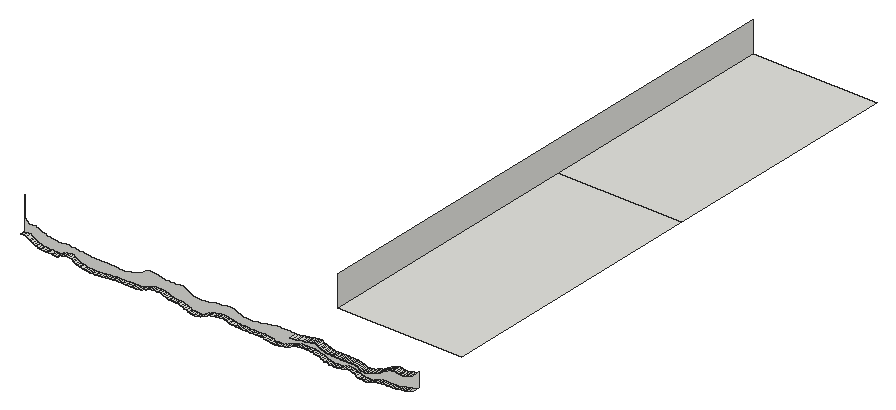
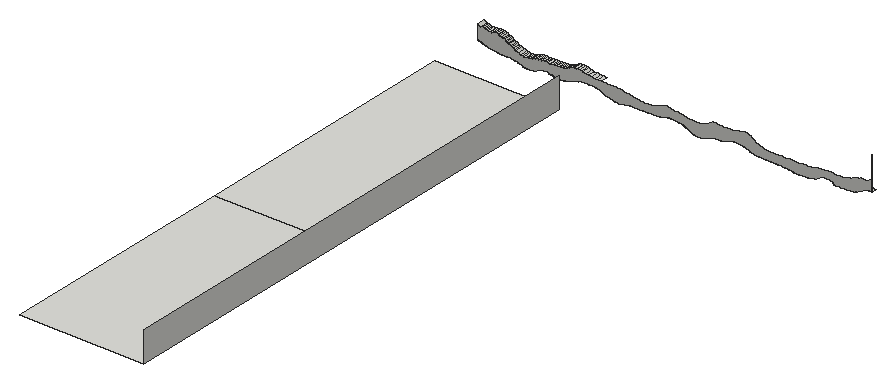
# SketchUp Ruby script. Lengths in inches.
U = 1.inch
M = Sketchup.active_model
def pt(a) = Geom::Point3d.new(a.map { |v| v * U })
def face(e, loops, mat)
  f = e.add_face(loops[0].map { |a| pt(a) })
  loops[1..].each { |l| e.add_face(l.map { |a| pt(a) }).erase! }
  f.material = f.back_material = mat if mat
  f
end
# faces: each face lists its corners as indices into pts; further lists are holes
def faces(e, pts, list, mat = nil) = list.each { |f| face(e, (f[0].is_a?(Array) ? f : [f]).map { |l| l.map { |i| pts[i] } }, mat) }
# xy, xz, yz: faces in a plane at the given z, y or x. An outline is a flat list of corners, or four numbers for a rectangle; further outlines are holes
def ring(l) = l.size == 4 ? [[l[0], l[1]], [l[2], l[1]], [l[2], l[3]], [l[0], l[3]]] : l.each_slice(2).to_a
def flat(e, list, mat, &to3) = list.each { |f| face(e, (f[0].is_a?(Array) ? f : [f]).map { |l| ring(l).map { |u, v| to3.(u, v) } }, mat) }
def xy(e, z, list, mat = nil) = flat(e, list, mat) { |x, y| [x, y, z] }
def xz(e, y, list, mat = nil) = flat(e, list, mat) { |x, z| [x, y, z] }
def yz(e, x, list, mat = nil) = flat(e, list, mat) { |y, z| [x, y, z] }
def lines(e, pts, list) = list.each { |a, b| e.add_line(pt(pts[a]), pt(pts[b])) }
# prism: a flat outline (further loops are holes) pulled along v
def prism(e, loops, v, mat = nil)
  f = face(e, loops, mat); d = Geom::Vector3d.new(v.map { |x| x * U })
  f.pushpull(f.normal.samedirection?(d) ? d.length : -d.length)
end
def box(e, o, s, mat = nil) = prism(e, [[o, [o[0] + s[0], o[1], o[2]], [o[0] + s[0], o[1] + s[1], o[2]], [o[0], o[1] + s[1], o[2]]]], [0, 0, s[2]], mat)
def at(x, y, z, deg = 0) = Geom::Transformation.translation(pt([x, y, z])) * Geom::Transformation.rotation(ORIGIN, Z_AXIS, deg.degrees)
def axes(o, x, y, z) = Geom::Transformation.new([*x, 0, *y, 0, *z, 0, *pt(o).to_a, 1])
def part(name) = M.definitions.add(name)
# library, detail: a bought-in or finely detailed component or shape, given as its bounding box
def library(name, o, s) = part(name).tap { |d| box(d.entities, o, s) }
def detail(e, o, s) = box(e.add_group.entities, o, s)
def put(e, d, t, mat = nil) = e.add_instance(d, t).tap { |i| i.material = mat if mat }
def group(e, t, mat = nil) = e.add_group.tap { |g| g.transformation = t; g.material = mat if mat }.entities
root = M.entities
xy(root,237.65,[[282.08,2402.3,282.77,2404.3],[282.77,2402.3,283.39,2404.3]])
xy(root,238.18,[[376.03,2402.3,376.71,2404.3]])
xy(root,238.33,[[291.18,2402.3,291.73,2404.3],[291.73,2402.3,292.41,2404.3]])
xy(root,238.34,[[293.09,2402.3,294.02,2404.3],[294.02,2402.3,294.51,2404.3],[294.51,2402.3,295.27,2404.3],[295.27,2402.3,295.9,2404.3],[295.9,2402.3,296.65,2404.3],
  [296.65,2402.3,297.27,2404.3],[297.27,2402.3,298.04,2404.3],[298.04,2402.3,298.66,2404.3]])
xy(root,238.62,[[342.56,2402.3,343.33,2404.3],[343.33,2402.3,343.96,2404.3],[343.96,2402.3,344.72,2404.3],[344.72,2402.3,345.34,2404.3],[345.34,2402.3,346.19,2404.3],
  [346.19,2402.3,346.83,2404.3],[346.83,2402.3,347.45,2404.3]])
xy(root,238.625,[[341.14,2402.3,342,2404.3]])
xy(root,238.89,[[396.95,2402.3,397.63,2404.3]])
xy(root,238.9,[[398.39,2402.3,399.01,2404.3],[399.01,2402.3,399.78,2404.3]])
xy(root,240.43,[[365.23,2402.3,365.8,2404.3]])
xy(root,241.52,[[252.78,2402.3,252.84,2404.3]])
xy(root,242.28,[[383.05,2401.37,383.5625,2404.3]])
xy(root,242.3,[[381.29,2401.37,381.96,2404.3]])
xy(root,242.33,[[378.88,2401.37,379.46,2404.3]])
xy(root,242.625,[[358.39,2425.46,406.85,2532.83],[358.39,2532.83,406.85,2628.15]])
xz(root,2404.3,[[321.7,236.98,321.09,237.01,320.4,237.04,319.64,237.11,318.95,237.2,318.42,237.33,317.75,237.68,316.8125,237.96,316.25,238.28,315.47,238.43,314.69,238.78,314.02,238.79,313.48,238.8,312.72,238.83,311.97,238.875,311.4,238.94,310.82,239.04,310.16,239.29,309.58,239.53,309.05,239.7,308.36,239.92,307.73,240.11,306.95,240.27,306.33,240.25,305.625,240.23,304.86,240.19,304.1875,240.12,303.53,240.03,302.89,239.85,302.34,239.52,301.78,239.35,301.19,239.18,300.68,238.86,299.99,238.72,299.17,238.59,298.66,238.34,293.09,238.34,292.41,238.33,291.18,238.33,290.46,238.32,289.61,238.3,288.98,238.28,288.23,238.26,287.6,238.15,286.84,238.13,286.29,238.1,285.4375,237.98,284.82,237.94,284.06,237.89,283.39,237.65,282.08,237.65,281.39,237.66,280.64,237.67,280.04,237.68,279.43,237.71,278.72,237.76,278.03,237.82,277.37,237.9,276.43,238.21,275.96,238.31,275.05,238.43,274.4,238.74,273.82,239.11,273.24,239.38,272.78,239.71,272.08,240.11,271.39,240.09,270.73,240.05,270.14,239.99,269.41,239.88,268.86,239.69,268.28,239.55,267.72,238.9375,267.19,238.77,266.45,238.79,265.58,238.8,265.07,238.82,264.03,238.92,263.34,238.93,262.64,238.94,261.94,238.97,261.26,239.03,260.57,239.09,259.79,239.19,259.28,239.52,258.72,239.64,258.27,239.86,257.48,240.2,256.88,240.59,256.34,240.85,255.32,241.55,254.05,241.69,252.84,241.52,252.84,246.2,254.41,244.96,255.8,244.9375,257.05,244.92,257.27,244.61,257.83,244.54,258.59,244.41,259.26,244.11,259.78,243.95,260.44,243.79,260.96,243.48,261.6,243.3,262.1875,243.14,262.67,243.06,263.39,242.85,263.97,242.78,264.78,242.73,265.32,242.68,265.99,242.51,266.51,242.46,267.05,242.58,267.68,242.57,268.31,242.81,268.88,242.86,269.44,242.89,270.08,242.92,270.51,242.625,271.12,242.65,271.67,242.62,272.3,242.58,272.86,242.57,273.5,242.48,274.16,242.38,274.82,242.34,275.49,242.24,276.66,241.96,277.43,241.89,278.25,241.83,278.85,241.78,279.62,241.75,280.07,241.74,280.62,241.72,281.88,241.7,282.61,241.69,283.28,241.68,283.87,241.68,284.36,241.67,285.0625,241.74,285.63,241.75,287.63,241.75,288.12,241.67,288.65,241.66,289.26,241.57,289.8,241.53,290.42,241.51,290.97,241.49,291.67,241.48,292.33,241.47,292.9,241.46,293.61,241.6,294.34,241.85,295.01,241.91,295.91,242.1,296.68,242.46,297.38,242.78,298.15,242.97,298.68,243.23,299.08,243.48,299.6,243.72,299.9375,244.12,300.41,244.39,300.89,244.73,301.375,244.87,301.96,244.95,302.64,245.01,303.29,244.81,303.86,244.7,304.34,244.67,304.95,244.55,305.49,244.51,305.95,244.25,306.7,244.11,307.26,244.04,307.88,243.99,308.6,243.95,309.1,243.93,309.79,243.91,310.36,243.89,311.06,243.88,311.71,243.94,312.35,243.95,312.91,244.1,313.54,244.13,314.02,244.15,314.54,244.17,315.06,244.18,315.66,243.8,316.2,243.43,316.81,243.09,317.2,242.875,317.7,242.68,318.29,242.51,318.8,242.21,319.4,242.11,320.08,241.96,320.64,241.89,321.1,241.85,321.62,241.8125,322.13,241.79,322.71,241.78,323.38,241.91,323.85,241.93,324.52,242.09,325.29,242.2,325.79,242.24,326.4,242.42,326.95,242.47,327.7,242.71,328.34,242.78,328.82,242.82,329.51,242.85,330.21,242.87,330.76,243.02,331.38,243.05,331.93,243.29,332.61,243.35,333.16,243.39,333.76,243.42,334.53,243.14,335.1,242.9375,335.65,242.65,336.27,242.39,337.03,242.14,337.67,241.89,338.16,241.78,339.21,241.63,339.98,241.56,340.58,241.51,341.03,241.48,341.55,241.46,342.42,241.51,343.14,241.59,344.08,241.82,344.86,241.87,345.625,241.98,346.24,242.02,346.89,242.19,347.59,242.38,348.08,242.4375,348.6,242.48,349.26,242.58,349.79,242.61,350.375,242.77,350.83,242.95,351.39,243.01,351.9,243.05,352.47,243.08,353.125,243.09,355.28,243.09,355.85,243.08,356.4375,243.07,357.02,243.07,357.68,243.0625,358.29,243.05,358.97,243.05,360.24,243.1,361.41,243.17,362.55,243.4,363.8125,243.52,364.94,243.71,365.84,243.99,366.54,244.08,367.24,244.21,367.82,244.27,368.36,244.3,369.03,244.39,369.625,244.19,370,243.88,370.48,243.59,371.03,243.33,371.58,243.22,372.07,242.92,372.55,242.75,373.11,242.6,373.67,242.52,374.23,242.47,374.8125,242.43,375.39,242.4,375.97,242.39,376.55,242.37,377.13,242.36,377.72,242.35,378.88,242.33,379.46,242.33,380.18,242.32,380.65,242.3125,381.29,242.3,381.96,242.3,382.41,242.29,383.05,242.28,383.5625,242.28,384.19,242.2,384.77,241.97,385.34,241.84,385.85,241.57,386.27,241.33,386.74,241.24,387.27,241.17,387.74,241.12,388.34,241.09,388.91,241.14,389.55,241.35,390.14,241.46,391.08,241.85,392.08,242.23,392.64,242.42,393.36,242.61,393.875,242.91,394.25,243.14,394.79,243.52,395.27,243.71,395.6,244.02,396.04,244.21,396.63,244.57,397.1,244.76,397.72,245.125,398.22,245.32,398.7,245.41,399.25,245.48,399.74,245.59,400.27,245.55,400.88,245.35,401.37,245.31,401.92,245.27,402.48,245.24,403.04,245.22,403.6,245.34,404.23,245.42,404.8125,245.52,405.19,245.76,405.66,245.9,406.85,246.43,406.85,240.89,405.02,240.1,404.46,239.96,403.9375,239.81,403.25,239.53,402.7,239.49,401.98,239.42,401.18,239.28,400.41,239.15,399.78,238.9,398.39,238.9,397.63,238.89,396.95,238.89,396.27,238.88,395.73,238.875,394.97,238.86,394.23,238.83,393.66,238.8,393.08,238.74,392.42,238.6,391.85,238.51,391.32,238.33,390.63,238.08,389.95,237.84,389.26,237.5625,388.66,237.47,387.98,237.4,387.25,237.42,386.68,237.45,386.09,237.51,385.49,237.59,384.95,237.71,384.12,238,383.41,238.33,382.86,238.57,382.36,238.86,381.84,238.96,381.15,239.02,380.47,239.125,379.73,239.04,379.16,238.66,378.57,238.61,377.91,238.55,377.39,238.27,376.71,238.18,376.03,238.18,375.36,238.11,374.83,238.15,374.01,238.19,373.4375,238.26,372.87,238.48,372.21,238.56,371.64,238.67,371.12,239.01,370.4375,239.18,369.8125,239.5,369.05,239.65,368.4375,239.8,367.68,239.96,367.03,240.23,366.45,240.27,365.8,240.43,365.23,240.43,364.65,240.42,364.125,240.41,363.43,240.4,362.74,240.37,362.05,240.33,361.37,240.27,360.69,240.17,360.07,239.97,359.42,239.75,358.68,239.375,357.89,239.08,357.01,238.72,356.26,238.46,355.04,238.14,353.92,237.88,353.27,237.87,352.4,237.74,351.69,237.79,350.92,237.86,350.29,238.15,349.52,238.19,348.9,238.25,348.14,238.45,347.45,238.62,342.56,238.62,342,238.625,341.14,238.625,340.45,238.63,339.83,238.64,339.05,238.65,338.38,238.66,337.69,238.6875,337.02,238.73,336.54,238.78,335.66,238.93,334.89,239.07,334.34,239.16,333.49,239.44,332.82,239.56,332.21,239.72,331.48,239.7,330.92,239.69,330.33,239.65,329.71,239.6,329.22,239.54,328.41,239.31,327.41,239.22,326.83,239.12,326.1875,238.76,325.55,238.51,324.99,238.375,324.55,238.02,323.85,237.74,323.23,237.43,322.38,237.22],[252.78,241.52,252.84,254.5]])
yz(root,358.39,[[2425.46,242.625,2628.15,254.5]])
p = [[319.64,2404.3,237.11],[320.4,2404.3,237.04],[320.4,2402.3,237.04],[319.64,2402.3,237.11],[321.09,2404.3,237.01],[321.09,2402.3,237.01],
  [321.7,2404.3,236.98],[321.7,2402.3,236.98],[322.38,2404.3,237.22],[322.38,2402.3,237.22],[318.95,2404.3,237.2],[318.95,2402.3,237.2],
  [318.42,2404.3,237.33],[318.42,2402.3,237.33],[323.23,2404.3,237.43],[323.23,2402.3,237.43],[317.75,2404.3,237.68],[317.75,2402.3,237.68],
  [323.85,2404.3,237.74],[323.85,2402.3,237.74],[386.68,2404.3,237.45],[387.25,2404.3,237.42],[387.25,2402.3,237.42],[386.68,2402.3,237.45],
  [387.98,2404.3,237.4],[387.98,2402.3,237.4],[388.66,2404.3,237.47],[388.66,2402.3,237.47],[385.49,2404.3,237.59],[386.09,2404.3,237.51],
  [386.09,2402.3,237.51],[385.49,2402.3,237.59],[389.26,2404.3,237.5625],[389.26,2402.3,237.5625],[283.39,2404.3,237.65],[284.06,2404.3,237.89],
  [284.06,2402.3,237.89],[283.39,2402.3,237.65],[384.95,2404.3,237.71],[384.95,2402.3,237.71],[389.95,2404.3,237.84],[389.95,2402.3,237.84],
  [278.72,2404.3,237.76],[279.43,2404.3,237.71],[279.43,2402.3,237.71],[278.72,2402.3,237.76],[280.04,2404.3,237.68],[280.04,2402.3,237.68],
  [280.64,2404.3,237.67],[280.64,2402.3,237.67],[281.39,2404.3,237.66],[281.39,2402.3,237.66],[282.08,2404.3,237.65],[282.08,2402.3,237.65],
  [316.8125,2404.3,237.96],[316.8125,2402.3,237.96],[324.55,2404.3,238.02],[324.55,2402.3,238.02],[351.69,2404.3,237.79],[352.4,2404.3,237.74],
  [352.4,2402.3,237.74],[351.69,2402.3,237.79],[353.27,2404.3,237.87],[353.27,2402.3,237.87],[384.12,2404.3,238],[384.12,2402.3,238],
  [277.37,2404.3,237.9],[278.03,2404.3,237.82],[278.03,2402.3,237.82],[277.37,2402.3,237.9],[350.92,2404.3,237.86],[350.92,2402.3,237.86],
  [390.63,2404.3,238.08],[390.63,2402.3,238.08],[276.43,2404.3,238.21],[276.43,2402.3,238.21],[284.82,2404.3,237.94],[284.82,2402.3,237.94],
  [285.4375,2404.3,237.98],[285.4375,2402.3,237.98],[350.29,2404.3,238.15],[350.29,2402.3,238.15],[353.92,2404.3,237.88],[353.92,2402.3,237.88],
  [355.04,2404.3,238.14],[355.04,2402.3,238.14],[286.29,2404.3,238.1],[286.29,2402.3,238.1],[316.25,2404.3,238.28],[316.25,2402.3,238.28],
  [324.99,2404.3,238.375],[324.99,2402.3,238.375],[383.41,2404.3,238.33],[383.41,2402.3,238.33],[286.84,2404.3,238.13],[286.84,2402.3,238.13],
  [287.6,2404.3,238.15],[287.6,2402.3,238.15],[349.52,2404.3,238.19],[349.52,2402.3,238.19],[356.26,2404.3,238.46],[356.26,2402.3,238.46],
  [374.01,2404.3,238.19],[374.83,2404.3,238.15],[374.83,2402.3,238.15],[374.01,2402.3,238.19],[375.36,2404.3,238.11],[375.36,2402.3,238.11],
  [376.03,2404.3,238.18],[376.03,2402.3,238.18],[391.32,2404.3,238.33],[391.32,2402.3,238.33],[275.96,2404.3,238.31],[275.96,2402.3,238.31],
  [288.23,2404.3,238.26],[288.23,2402.3,238.26],[348.9,2404.3,238.25],[348.9,2402.3,238.25],[373.4375,2404.3,238.26],[373.4375,2402.3,238.26],
  [376.71,2404.3,238.18],[377.39,2404.3,238.27],[377.39,2402.3,238.27],[376.71,2402.3,238.18],[275.05,2404.3,238.43],[275.05,2402.3,238.43],
  [288.98,2404.3,238.28],[288.98,2402.3,238.28],[289.61,2404.3,238.3],[289.61,2402.3,238.3],[290.46,2404.3,238.32],[290.46,2402.3,238.32],
  [291.18,2404.3,238.33],[291.18,2402.3,238.33],[292.41,2404.3,238.33],[293.09,2404.3,238.34],[293.09,2402.3,238.34],[292.41,2402.3,238.33],
  [298.66,2404.3,238.34],[299.17,2404.3,238.59],[299.17,2402.3,238.59],[298.66,2402.3,238.34],[315.47,2404.3,238.43],[315.47,2402.3,238.43],
  [348.14,2404.3,238.45],[348.14,2402.3,238.45],[372.87,2404.3,238.48],[372.87,2402.3,238.48],[377.91,2404.3,238.55],[377.91,2402.3,238.55],
  [382.86,2404.3,238.57],[382.86,2402.3,238.57],[391.85,2404.3,238.51],[391.85,2402.3,238.51],[274.4,2404.3,238.74],[274.4,2402.3,238.74],
  [314.69,2404.3,238.78],[314.69,2402.3,238.78],[325.55,2404.3,238.51],[325.55,2402.3,238.51],[326.1875,2404.3,238.76],[326.1875,2402.3,238.76],
  [347.45,2404.3,238.62],[347.45,2402.3,238.62],[357.01,2404.3,238.72],[357.01,2402.3,238.72],[372.21,2404.3,238.56],[372.21,2402.3,238.56],
  [378.57,2404.3,238.61],[378.57,2402.3,238.61],[392.42,2404.3,238.6],[392.42,2402.3,238.6],[299.99,2404.3,238.72],[299.99,2402.3,238.72],
  [338.38,2404.3,238.66],[339.05,2404.3,238.65],[339.05,2402.3,238.65],[338.38,2402.3,238.66],[339.83,2404.3,238.64],[339.83,2402.3,238.64],
  [340.45,2404.3,238.63],[340.45,2402.3,238.63],[341.14,2404.3,238.625],[341.14,2402.3,238.625],[342,2404.3,238.625],[342.56,2404.3,238.62],
  [342.56,2402.3,238.62],[342,2402.3,238.625],[371.64,2404.3,238.67],[371.64,2402.3,238.67],[379.16,2404.3,238.66],[379.16,2402.3,238.66],
  [382.36,2404.3,238.86],[382.36,2402.3,238.86],[393.08,2404.3,238.74],[393.08,2402.3,238.74],[273.82,2404.3,239.11],[273.82,2402.3,239.11],
  [300.68,2404.3,238.86],[300.68,2402.3,238.86],[336.54,2404.3,238.78],[337.02,2404.3,238.73],[337.02,2402.3,238.73],[336.54,2402.3,238.78],
  [337.69,2404.3,238.6875],[337.69,2402.3,238.6875],[357.89,2404.3,239.08],[357.89,2402.3,239.08],[371.12,2404.3,239.01],[371.12,2402.3,239.01],
  [379.73,2404.3,239.04],[379.73,2402.3,239.04],[393.66,2404.3,238.8],[393.66,2402.3,238.8],[264.03,2404.3,238.92],[265.07,2404.3,238.82],
  [265.07,2402.3,238.82],[264.03,2402.3,238.92],[265.58,2404.3,238.8],[265.58,2402.3,238.8],[266.45,2404.3,238.79],[266.45,2402.3,238.79],
  [267.19,2404.3,238.77],[267.19,2402.3,238.77],[267.72,2404.3,238.9375],[267.72,2402.3,238.9375],[311.97,2404.3,238.875],[312.72,2404.3,238.83],
  [312.72,2402.3,238.83],[311.97,2402.3,238.875],[313.48,2404.3,238.8],[313.48,2402.3,238.8],[314.02,2404.3,238.79],[314.02,2402.3,238.79],
  [326.83,2404.3,239.12],[326.83,2402.3,239.12],[335.66,2404.3,238.93],[335.66,2402.3,238.93],[394.23,2404.3,238.83],[394.23,2402.3,238.83],
  [394.97,2404.3,238.86],[394.97,2402.3,238.86],[261.94,2404.3,238.97],[262.64,2404.3,238.94],[262.64,2402.3,238.94],[261.94,2402.3,238.97],
  [263.34,2404.3,238.93],[263.34,2402.3,238.93],[268.28,2404.3,239.55],[268.28,2402.3,239.55],[301.19,2404.3,239.18],[301.19,2402.3,239.18],
  [310.82,2404.3,239.04],[311.4,2404.3,238.94],[311.4,2402.3,238.94],[310.82,2402.3,239.04],[334.89,2404.3,239.07],[334.89,2402.3,239.07],
  [381.84,2404.3,238.96],[381.84,2402.3,238.96],[395.73,2404.3,238.875],[395.73,2402.3,238.875],[396.27,2404.3,238.88],[396.27,2402.3,238.88],
  [396.95,2404.3,238.89],[396.95,2402.3,238.89],[397.63,2404.3,238.89],[398.39,2404.3,238.9],[398.39,2402.3,238.9],[397.63,2402.3,238.89],
  [399.78,2404.3,238.9],[400.41,2404.3,239.15],[400.41,2402.3,239.15],[399.78,2402.3,238.9],[260.57,2404.3,239.09],[261.26,2404.3,239.03],
  [261.26,2402.3,239.03],[260.57,2402.3,239.09],[310.16,2404.3,239.29],[310.16,2402.3,239.29],[370.4375,2404.3,239.18],[370.4375,2402.3,239.18],
  [380.47,2404.3,239.125],[380.47,2402.3,239.125],[381.15,2404.3,239.02],[381.15,2402.3,239.02],[259.79,2404.3,239.19],[259.79,2402.3,239.19],
  [273.24,2404.3,239.38],[273.24,2402.3,239.38],[327.41,2404.3,239.22],[327.41,2402.3,239.22],[334.34,2404.3,239.16],[334.34,2402.3,239.16],
  [358.68,2404.3,239.375],[358.68,2402.3,239.375],[259.28,2404.3,239.52],[259.28,2402.3,239.52],[301.78,2404.3,239.35],[301.78,2402.3,239.35],
  [328.41,2404.3,239.31],[328.41,2402.3,239.31],[333.49,2404.3,239.44],[333.49,2402.3,239.44],[369.8125,2404.3,239.5],[369.8125,2402.3,239.5],
  [401.18,2404.3,239.28],[401.18,2402.3,239.28],[309.58,2404.3,239.53],[309.58,2402.3,239.53],[329.22,2404.3,239.54],[329.22,2402.3,239.54],
  [401.98,2404.3,239.42],[401.98,2402.3,239.42],[272.78,2404.3,239.71],[272.78,2402.3,239.71],[302.34,2404.3,239.52],[302.34,2402.3,239.52],
  [332.82,2404.3,239.56],[332.82,2402.3,239.56],[359.42,2404.3,239.75],[359.42,2402.3,239.75],[402.7,2404.3,239.49],[402.7,2402.3,239.49],
  [258.72,2404.3,239.64],[258.72,2402.3,239.64],[302.89,2404.3,239.85],[302.89,2402.3,239.85],[309.05,2404.3,239.7],[309.05,2402.3,239.7],
  [329.71,2404.3,239.6],[329.71,2402.3,239.6],[369.05,2404.3,239.65],[369.05,2402.3,239.65],[403.25,2404.3,239.53],[403.25,2402.3,239.53],
  [403.9375,2404.3,239.81],[403.9375,2402.3,239.81],[258.27,2404.3,239.86],[258.27,2402.3,239.86],[268.86,2404.3,239.69],[268.86,2402.3,239.69],
  [330.33,2404.3,239.65],[330.33,2402.3,239.65],[330.92,2404.3,239.69],[330.92,2402.3,239.69],[332.21,2404.3,239.72],[332.21,2402.3,239.72],
  [269.41,2404.3,239.88],[269.41,2402.3,239.88],[272.08,2404.3,240.11],[272.08,2402.3,240.11],[308.36,2404.3,239.92],[308.36,2402.3,239.92],
  [331.48,2404.3,239.7],[331.48,2402.3,239.7],[360.07,2404.3,239.97],[360.07,2402.3,239.97],[368.4375,2404.3,239.8],[368.4375,2402.3,239.8],
  [303.53,2404.3,240.03],[303.53,2402.3,240.03],[367.68,2404.3,239.96],[367.68,2402.3,239.96],[404.46,2404.3,239.96],[404.46,2402.3,239.96],
  [257.48,2404.3,240.2],[257.48,2402.3,240.2],[270.14,2404.3,239.99],[270.14,2402.3,239.99],[307.73,2404.3,240.11],[307.73,2402.3,240.11],
  [270.73,2404.3,240.05],[270.73,2402.3,240.05],[271.39,2404.3,240.09],[271.39,2402.3,240.09],[304.1875,2404.3,240.12],[304.1875,2402.3,240.12],
  [360.69,2404.3,240.17],[360.69,2402.3,240.17],[367.03,2404.3,240.23],[367.03,2402.3,240.23],[405.02,2404.3,240.1],[405.02,2402.3,240.1],
  [304.86,2404.3,240.19],[304.86,2402.3,240.19],[306.95,2404.3,240.27],[306.95,2402.3,240.27],[406.85,2404.3,240.89],[406.85,2402.3,240.89],
  [256.88,2404.3,240.59],[256.88,2402.3,240.59],[305.625,2404.3,240.23],[305.625,2402.3,240.23],[306.33,2404.3,240.25],[306.33,2402.3,240.25],
  [361.37,2404.3,240.27],[361.37,2402.3,240.27],[366.45,2404.3,240.27],[366.45,2402.3,240.27],[362.05,2404.3,240.33],[362.05,2402.3,240.33],
  [362.74,2404.3,240.37],[362.74,2402.3,240.37],[365.8,2404.3,240.43],[365.8,2402.3,240.43],[363.43,2404.3,240.4],[363.43,2402.3,240.4],
  [364.125,2404.3,240.41],[364.125,2402.3,240.41],[364.65,2404.3,240.42],[364.65,2402.3,240.42],[365.23,2404.3,240.43],[365.23,2402.3,240.43],
  [256.34,2404.3,240.85],[256.34,2402.3,240.85],[255.32,2404.3,241.55],[255.32,2402.3,241.55],[387.27,2404.3,241.17],[387.74,2404.3,241.12],
  [387.74,2401.37,241.12],[387.27,2401.37,241.17],[388.34,2404.3,241.09],[388.34,2401.37,241.09],[388.91,2404.3,241.14],[388.91,2401.37,241.14],
  [389.55,2404.3,241.35],[389.55,2401.37,241.35],[386.27,2404.3,241.33],[386.74,2404.3,241.24],[386.74,2401.37,241.24],[386.27,2401.37,241.33],
  [385.85,2404.3,241.57],[385.85,2401.37,241.57],[390.14,2404.3,241.46],[390.14,2401.37,241.46],[391.08,2404.3,241.85],[391.08,2401.37,241.85],
  [252.84,2404.3,241.52],[254.05,2404.3,241.69],[254.05,2402.3,241.69],[252.84,2402.3,241.52],[385.34,2404.3,241.84],[385.34,2401.37,241.84],
  [384.77,2404.3,241.97],[384.77,2401.37,241.97],[392.08,2404.3,242.23],[392.08,2401.37,242.23],[384.19,2404.3,242.2],[384.19,2401.37,242.2],
  [383.5625,2404.3,242.28],[383.5625,2401.37,242.28],[392.64,2404.3,242.42],[392.64,2401.37,242.42],[377.72,2404.3,242.35],[378.3,2404.3,242.34],
  [378.3,2401.37,242.34],[377.72,2401.37,242.35],[378.88,2404.3,242.33],[378.88,2401.37,242.33],[379.46,2404.3,242.33],[380.18,2404.3,242.32],
  [380.18,2401.37,242.32],[379.46,2401.37,242.33],[380.65,2404.3,242.3125],[380.65,2401.37,242.3125],[381.29,2404.3,242.3],[381.29,2401.37,242.3],
  [381.96,2404.3,242.3],[382.41,2404.3,242.29],[382.41,2401.37,242.29],[381.96,2401.37,242.3],[383.05,2404.3,242.28],[383.05,2401.37,242.28],
  [374.23,2404.3,242.47],[374.8125,2404.3,242.43],[374.8125,2401.37,242.43],[374.23,2401.37,242.47],[375.39,2404.3,242.4],[375.39,2401.37,242.4],
  [375.97,2404.3,242.39],[375.97,2401.37,242.39],[376.55,2404.3,242.37],[376.55,2401.37,242.37],[377.13,2404.3,242.36],[377.13,2401.37,242.36],
  [393.36,2404.3,242.61],[393.36,2401.37,242.61],[373.11,2404.3,242.6],[373.67,2404.3,242.52],[373.67,2401.37,242.52],[373.11,2401.37,242.6],
  [372.55,2404.3,242.75],[372.55,2401.37,242.75],[393.875,2404.3,242.91],[393.875,2401.37,242.91],[372.07,2404.3,242.92],[372.07,2401.37,242.92],
  [371.58,2404.3,243.22],[371.58,2401.37,243.22],[394.25,2404.3,243.14],[394.25,2401.37,243.14],[358.97,2404.3,243.05],[360.24,2404.3,243.1],
  [360.24,2401.37,243.1],[358.97,2401.37,243.05],[361.41,2404.3,243.17],[361.41,2401.37,243.17],[394.79,2404.3,243.52],[394.79,2401.37,243.52],
  [362.55,2404.3,243.4],[362.55,2401.37,243.4],[371.03,2404.3,243.33],[371.03,2401.37,243.33],[370.48,2404.3,243.59],[370.48,2401.37,243.59],
  [363.8125,2404.3,243.52],[363.8125,2401.37,243.52],[364.94,2404.3,243.71],[364.94,2401.37,243.71],[395.27,2404.3,243.71],[395.27,2401.37,243.71],
  [370,2404.3,243.88],[370,2401.37,243.88],[365.84,2404.3,243.99],[365.84,2401.37,243.99],[395.6,2404.3,244.02],[395.6,2401.37,244.02],
  [369.625,2404.3,244.19],[369.625,2401.37,244.19],[366.54,2404.3,244.08],[366.54,2401.37,244.08],[396.04,2404.3,244.21],[396.04,2401.37,244.21],
  [367.24,2404.3,244.21],[367.24,2401.37,244.21],[367.82,2404.3,244.27],[367.82,2401.37,244.27],[369.03,2404.3,244.39],[369.03,2401.37,244.39],
  [396.63,2404.3,244.57],[396.63,2401.37,244.57],[368.36,2404.3,244.3],[368.36,2401.37,244.3],[397.1,2404.3,244.76],[397.1,2401.37,244.76],
  [397.72,2404.3,245.125],[397.72,2401.37,245.125],[398.22,2404.3,245.32],[398.22,2401.37,245.32],[401.92,2404.3,245.27],[402.48,2404.3,245.24],
  [402.48,2401.37,245.24],[401.92,2401.37,245.27],[403.04,2404.3,245.22],[403.04,2401.37,245.22],[403.6,2404.3,245.34],[403.6,2401.37,245.34],
  [398.7,2404.3,245.41],[398.7,2401.37,245.41],[400.27,2404.3,245.55],[400.88,2404.3,245.35],[400.88,2401.37,245.35],[400.27,2401.37,245.55],
  [401.37,2404.3,245.31],[401.37,2401.37,245.31],[404.23,2404.3,245.42],[404.23,2401.37,245.42],[399.25,2404.3,245.48],[399.25,2401.37,245.48],
  [404.8125,2404.3,245.52],[404.8125,2401.37,245.52],[399.74,2404.3,245.59],[399.74,2401.37,245.59],[405.19,2404.3,245.76],[405.19,2401.37,245.76],
  [405.66,2404.3,245.9],[405.66,2401.37,245.9],[406.85,2404.3,246.43],[406.85,2401.37,246.43]]
faces(root,p,[[0,1,2,3],[1,4,5,2],[4,6,7,5],[6,8,9,7],[10,0,3,11],[12,10,11,13],[8,14,15,9],[16,12,13,17],
  [14,18,19,15],[20,21,22,23],[21,24,25,22],[24,26,27,25],[28,29,30,31],[29,20,23,30],[26,32,33,27],[34,35,36,37],
  [38,28,31,39],[32,40,41,33],[42,43,44,45],[43,46,47,44],[46,48,49,47],[48,50,51,49],[50,52,53,51],[54,16,17,55],
  [18,56,57,19],[58,59,60,61],[59,62,63,60],[64,38,39,65],[66,67,68,69],[67,42,45,68],[70,58,61,71],[40,72,73,41],
  [74,66,69,75],[35,76,77,36],[76,78,79,77],[80,70,71,81],[62,82,83,63],[82,84,85,83],[78,86,87,79],[88,54,55,89],
  [56,90,91,57],[92,64,65,93],[86,94,95,87],[94,96,97,95],[98,80,81,99],[84,100,101,85],[102,103,104,105],[103,106,107,104],
  [106,108,109,107],[72,110,111,73],[112,74,75,113],[96,114,115,97],[116,98,99,117],[118,102,105,119],[120,121,122,123],[124,112,113,125],
  [114,126,127,115],[126,128,129,127],[128,130,131,129],[130,132,133,131],[134,135,136,137],[138,139,140,141],[142,88,89,143],[144,116,117,145],
  [146,118,119,147],[121,148,149,122],[150,92,93,151],[110,152,153,111],[154,124,125,155],[156,142,143,157],[90,158,159,91],[158,160,161,159],
  [162,144,145,163],[100,164,165,101],[166,146,147,167],[148,168,169,149],[152,170,171,153],[139,172,173,140],[174,175,176,177],[175,178,179,176],
  [178,180,181,179],[180,182,183,181],[184,185,186,187],[188,166,167,189],[168,190,191,169],[192,150,151,193],[170,194,195,171],[196,154,155,197],
  [172,198,199,173],[200,201,202,203],[201,204,205,202],[204,174,177,205],[164,206,207,165],[208,188,189,209],[190,210,211,191],[194,212,213,195],
  [214,215,216,217],[215,218,219,216],[218,220,221,219],[220,222,223,221],[222,224,225,223],[226,227,228,229],[227,230,231,228],[230,232,233,231],
  [232,156,157,233],[160,234,235,161],[236,200,203,237],[212,238,239,213],[238,240,241,239],[242,243,244,245],[243,246,247,244],[246,214,217,247],
  [224,248,249,225],[198,250,251,199],[252,253,254,255],[253,226,229,254],[256,236,237,257],[258,192,193,259],[240,260,261,241],[260,262,263,261],
  [262,264,265,263],[266,267,268,269],[270,271,272,273],[274,275,276,277],[275,242,245,276],[278,252,255,279],[280,208,209,281],[210,282,283,211],
  [282,284,285,283],[284,258,259,285],[286,274,277,287],[288,196,197,289],[234,290,291,235],[292,256,257,293],[206,294,295,207],[296,286,287,297],
  [250,298,299,251],[290,300,301,291],[302,292,293,303],[304,280,281,305],[271,306,307,272],[308,278,279,309],[300,310,311,301],[306,312,313,307],
  [314,288,289,315],[298,316,317,299],[318,302,303,319],[294,320,321,295],[312,322,323,313],[324,296,297,325],[316,326,327,317],[328,308,309,329],
  [310,330,331,311],[332,304,305,333],[322,334,335,323],[334,336,337,335],[338,324,325,339],[248,340,341,249],[330,342,343,331],[342,344,345,343],
  [346,318,319,347],[340,348,349,341],[350,314,315,351],[352,328,329,353],[344,354,355,345],[354,346,347,355],[320,356,357,321],[358,332,333,359],
  [326,360,361,327],[362,358,359,363],[336,364,365,337],[366,338,339,367],[348,368,369,349],[370,352,353,371],[368,372,373,369],[372,374,375,373],
  [360,376,377,361],[356,378,379,357],[380,362,363,381],[364,382,383,365],[374,350,351,375],[376,384,385,377],[386,370,371,387],[382,388,389,383],
  [390,366,367,391],[384,392,393,385],[392,394,395,393],[378,396,397,379],[398,380,381,399],[394,386,387,395],[396,400,401,397],[400,402,403,401],
  [404,398,399,405],[402,406,407,403],[406,408,409,407],[408,410,411,409],[410,412,413,411],[414,390,391,415],[416,414,415,417],[418,419,420,421],
  [419,422,423,420],[422,424,425,423],[424,426,427,425],[428,429,430,431],[429,418,421,430],[432,428,431,433],[426,434,435,427],[434,436,437,435],
  [438,439,440,441],[442,432,433,443],[439,416,417,440],[444,442,443,445],[436,446,447,437],[448,444,445,449],[450,448,449,451],[446,452,453,447],
  [454,455,456,457],[455,458,459,456],[460,461,462,463],[461,464,465,462],[464,466,467,465],[468,469,470,471],[469,472,473,470],[474,475,476,477],
  [475,478,479,476],[478,480,481,479],[480,482,483,481],[482,484,485,483],[484,454,457,485],[452,486,487,453],[488,489,490,491],[489,474,477,490],
  [492,488,491,493],[486,494,495,487],[496,492,493,497],[498,496,497,499],[494,500,501,495],[502,503,504,505],[503,506,507,504],[500,508,509,501],
  [506,510,511,507],[512,498,499,513],[514,512,513,515],[510,516,517,511],[516,518,519,517],[508,520,521,509],[522,514,515,523],[518,524,525,519],
  [520,526,527,521],[528,522,523,529],[524,530,531,525],[526,532,533,527],[530,534,535,531],[534,536,537,535],[538,528,529,539],[532,540,541,533],
  [536,542,543,537],[542,538,539,543],[540,544,545,541],[544,546,547,545],[546,548,549,547],[550,551,552,553],[551,554,555,552],[554,556,557,555],
  [548,558,559,549],[560,561,562,563],[561,564,565,562],[564,550,553,565],[556,566,567,557],[558,568,569,559],[566,570,571,567],[568,572,573,569],
  [570,574,575,571],[572,560,563,573],[574,576,577,575],[576,578,579,577]])
